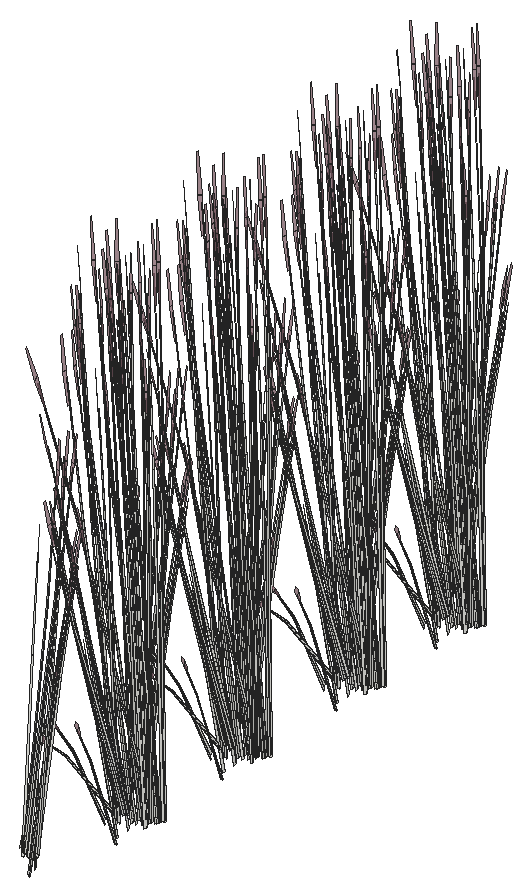
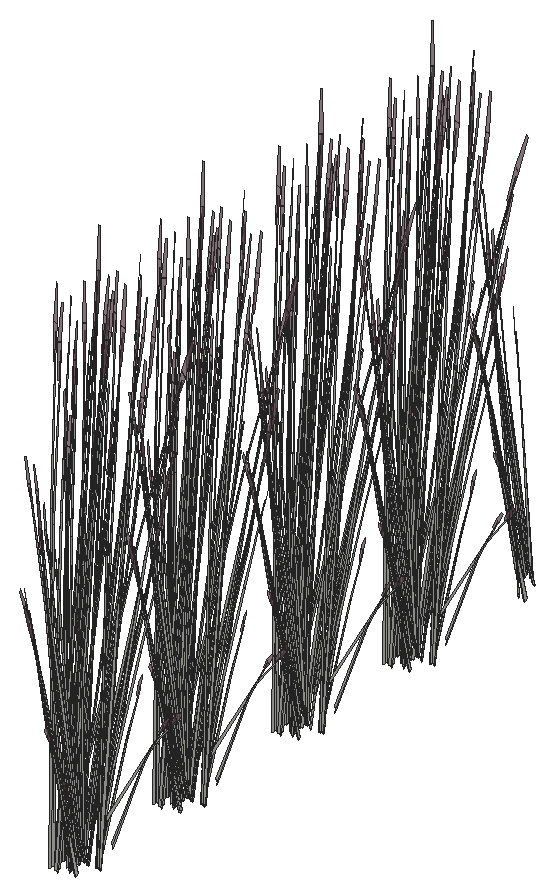
# SketchUp Ruby script. Lengths in inches.
U = 1.inch
M = Sketchup.active_model
def pt(a) = Geom::Point3d.new(a.map { |v| v * U })
def face(e, loops, mat)
  f = e.add_face(loops[0].map { |a| pt(a) })
  loops[1..].each { |l| e.add_face(l.map { |a| pt(a) }).erase! }
  f.material = f.back_material = mat if mat
  f
end
# faces: each face lists its corners as indices into pts; further lists are holes
def faces(e, pts, list, mat = nil) = list.each { |f| face(e, (f[0].is_a?(Array) ? f : [f]).map { |l| l.map { |i| pts[i] } }, mat) }
# xy, xz, yz: faces in a plane at the given z, y or x. An outline is a flat list of corners, or four numbers for a rectangle; further outlines are holes
def ring(l) = l.size == 4 ? [[l[0], l[1]], [l[2], l[1]], [l[2], l[3]], [l[0], l[3]]] : l.each_slice(2).to_a
def flat(e, list, mat, &to3) = list.each { |f| face(e, (f[0].is_a?(Array) ? f : [f]).map { |l| ring(l).map { |u, v| to3.(u, v) } }, mat) }
def xy(e, z, list, mat = nil) = flat(e, list, mat) { |x, y| [x, y, z] }
def xz(e, y, list, mat = nil) = flat(e, list, mat) { |x, z| [x, y, z] }
def yz(e, x, list, mat = nil) = flat(e, list, mat) { |y, z| [x, y, z] }
def lines(e, pts, list) = list.each { |a, b| e.add_line(pt(pts[a]), pt(pts[b])) }
# prism: a flat outline (further loops are holes) pulled along v
def prism(e, loops, v, mat = nil)
  f = face(e, loops, mat); d = Geom::Vector3d.new(v.map { |x| x * U })
  f.pushpull(f.normal.samedirection?(d) ? d.length : -d.length)
end
def box(e, o, s, mat = nil) = prism(e, [[o, [o[0] + s[0], o[1], o[2]], [o[0] + s[0], o[1] + s[1], o[2]], [o[0], o[1] + s[1], o[2]]]], [0, 0, s[2]], mat)
def at(x, y, z, deg = 0) = Geom::Transformation.translation(pt([x, y, z])) * Geom::Transformation.rotation(ORIGIN, Z_AXIS, deg.degrees)
def axes(o, x, y, z) = Geom::Transformation.new([*x, 0, *y, 0, *z, 0, *pt(o).to_a, 1])
def part(name) = M.definitions.add(name)
# library, detail: a bought-in or finely detailed component or shape, given as its bounding box
def library(name, o, s) = part(name).tap { |d| box(d.entities, o, s) }
def detail(e, o, s) = box(e.add_group.entities, o, s)
def put(e, d, t, mat = nil) = e.add_instance(d, t).tap { |i| i.material = mat if mat }
def group(e, t, mat = nil) = e.add_group.tap { |g| g.transformation = t; g.material = mat if mat }.entities
root = M.entities
M.materials.add("LightPink_Translucent").color = [144, 107, 117]
M.materials["LightPink_Translucent"].alpha = 0.75
c1 = part("blade")
p = [[2.15,0.21,22],[0,0.17,0],[0.09,0.45,0],[2.18,0.31,22],[2.29,0.31,22],[0.38,0.45,0],
  [2.48,0.24,33],[2.49,0.24,33],[2.48,0.22,33]]
faces(c1.entities,p,[[0,1,2,3],[4,5,2,3],[6,3,4,7],[8,0,3,6]])
c2 = part("seeds")
p = [[0.3,-0.1,1.38],[-0.01,-0.03,1.59],[-0.01,-0.03,0.03],[0.14,-0.07,-0.07],[0.29,-0.03,3],[0.15,0.01,3.11]]
faces(c2.entities,p,[[0,1,2,3],[1,0,4,5]],"LightPink_Translucent")
c3 = part("blade with seeds")
put(c3.entities,c1,at(0,0,0))
put(c3.entities,c2,axes([2.4,0.25,30.99],[1.5799,-0.05474,1.17369],[-0.12525,1.92788,0.29478],[-0.07173,-0.02425,1.56792]))
put(root,c3,axes([340.43,150.67,657.88],[-0.40605,-0.0193,0.05273],[0.01113,-0.29147,0.41509],[-0.04249,0.11165,0.63295]))
put(root,c3,axes([340.43,163.31,657.88],[-0.40605,-0.0193,0.05273],[0.01113,-0.29147,0.41509],[-0.04249,0.11165,0.63295]))
put(root,c3,axes([340.43,176.78,657.88],[-0.40605,-0.0193,0.05273],[0.01113,-0.29147,0.41509],[-0.04249,0.11165,0.63295]))
put(root,c3,axes([340.43,188.65,657.88],[-0.40605,-0.0193,0.05273],[0.01113,-0.29147,0.41509],[-0.04249,0.11165,0.63295]))
put(root,c3,axes([340.5625,137.6875,657.71],[-0.33433,0.21811,-0.29039],[-0.31649,-0.24905,0.3749],[-0.04815,0.12654,0.71734]))
put(root,c3,axes([340.5625,150.78,657.71],[-0.33433,0.21811,-0.29039],[-0.31649,-0.24905,0.3749],[-0.04815,0.12654,0.71734]))
put(root,c3,axes([340.5625,163.42,657.71],[-0.33433,0.21811,-0.29039],[-0.31649,-0.24905,0.3749],[-0.04815,0.12654,0.71734]))
put(root,c3,axes([340.5625,176.9,657.71],[-0.33433,0.21811,-0.29039],[-0.31649,-0.24905,0.3749],[-0.04815,0.12654,0.71734]))
put(root,c3,axes([340.5625,188.76,657.71],[-0.33433,0.21811,-0.29039],[-0.31649,-0.24905,0.3749],[-0.04815,0.12654,0.71734]))
put(root,c3,axes([342.27,150.13,655.6875],[-0.33282,0.31137,-0.51129],[-0.41344,-0.28235,-0.13419],[-0.13336,0.07767,1.12859]))
put(root,c3,axes([342.27,162.77,655.6875],[-0.33282,0.31137,-0.51129],[-0.41344,-0.28235,-0.13419],[-0.13336,0.07767,1.12859]))
put(root,c3,axes([342.27,176.24,655.6875],[-0.33282,0.31137,-0.51129],[-0.41344,-0.28235,-0.13419],[-0.13336,0.07767,1.12859]))
put(root,c3,axes([342.27,188.1,655.6875],[-0.33282,0.31137,-0.51129],[-0.41344,-0.28235,-0.13419],[-0.13336,0.07767,1.12859]))
put(root,c3,axes([341.42,147.81,658.14],[0.07631,0.33368,0.29039],[-0.43626,0.08811,-0.3749],[-0.11718,-0.09562,0.71734]))
put(root,c3,axes([341.42,160.45,658.14],[0.07631,0.33368,0.29039],[-0.43626,0.08811,-0.3749],[-0.11718,-0.09562,0.71734]))
put(root,c3,axes([341.42,173.93,658.14],[0.07631,0.33368,0.29039],[-0.43626,0.08811,-0.3749],[-0.11718,-0.09562,0.71734]))
put(root,c3,axes([341.42,185.79,658.14],[0.07631,0.33368,0.29039],[-0.43626,0.08811,-0.3749],[-0.11718,-0.09562,0.71734]))
put(root,c3,axes([339.37,138.46,657.86],[0.05606,-0.02501,1.45454],[0.46332,0.16636,-0.13744],[-0.01089,0.13852,0.2574]))
put(root,c3,axes([339.37,151.56,657.86],[0.05606,-0.02501,1.45454],[0.46332,0.16636,-0.13744],[-0.01089,0.13852,0.2574]))
put(root,c3,axes([339.37,164.19,657.86],[0.05606,-0.02501,1.45454],[0.46332,0.16636,-0.13744],[-0.01089,0.13852,0.2574]))
put(root,c3,axes([339.37,177.67,657.86],[0.05606,-0.02501,1.45454],[0.46332,0.16636,-0.13744],[-0.01089,0.13852,0.2574]))
put(root,c3,axes([339.37,189.53,657.86],[0.05606,-0.02501,1.45454],[0.46332,0.16636,-0.13744],[-0.01089,0.13852,0.2574]))
put(root,c3,axes([340.42,149.11,655.91],[-0.45961,0.34828,0.2522],[-0.45989,-0.34462,-0.29923],[-0.01605,-0.09891,1.35206]))
put(root,c3,axes([340.42,161.74,655.91],[-0.45961,0.34828,0.2522],[-0.45989,-0.34462,-0.29923],[-0.01605,-0.09891,1.35206]))
put(root,c3,axes([340.42,175.22,655.91],[-0.45961,0.34828,0.2522],[-0.45989,-0.34462,-0.29923],[-0.01605,-0.09891,1.35206]))
put(root,c3,axes([340.42,187.08,655.91],[-0.45961,0.34828,0.2522],[-0.45989,-0.34462,-0.29923],[-0.01605,-0.09891,1.35206]))
put(root,c3,axes([342.3125,150.07,656.73],[0.427,0.16705,1.24034],[-0.41831,0.35988,0.49049],[-0.18737,-0.21329,1.03981]))
put(root,c3,axes([342.3125,162.71,656.73],[0.427,0.16705,1.24034],[-0.41831,0.35988,0.49049],[-0.18737,-0.21329,1.03981]))
put(root,c3,axes([342.3125,176.18,656.73],[0.427,0.16705,1.24034],[-0.41831,0.35988,0.49049],[-0.18737,-0.21329,1.03981]))
put(root,c3,axes([342.3125,188.04,656.73],[0.427,0.16705,1.24034],[-0.41831,0.35988,0.49049],[-0.18737,-0.21329,1.03981]))
put(root,c3,axes([340.68,147.04,656.27],[0.25775,0.14418,0.94186],[-0.37538,0.08667,0.69201],[-0.08032,-0.11081,0.20745]))
put(root,c3,axes([340.68,159.68,656.27],[0.25775,0.14418,0.94186],[-0.37538,0.08667,0.69201],[-0.08032,-0.11081,0.20745]))
put(root,c3,axes([340.68,173.15,656.27],[0.25775,0.14418,0.94186],[-0.37538,0.08667,0.69201],[-0.08032,-0.11081,0.20745]))
put(root,c3,axes([340.68,185.02,656.27],[0.25775,0.14418,0.94186],[-0.37538,0.08667,0.69201],[-0.08032,-0.11081,0.20745]))
put(root,c3,axes([342.5,149.95,656.02],[-0.48249,-0.33343,-0.20658],[0.406,-0.37441,0.45206],[-0.12993,0.039,1.37937]))
put(root,c3,axes([342.5,162.59,656.02],[-0.48249,-0.33343,-0.20658],[0.406,-0.37441,0.45206],[-0.12993,0.039,1.37937]))
put(root,c3,axes([342.5,176.07,656.02],[-0.48249,-0.33343,-0.20658],[0.406,-0.37441,0.45206],[-0.12993,0.039,1.37937]))
put(root,c3,axes([342.5,187.93,656.02],[-0.48249,-0.33343,-0.20658],[0.406,-0.37441,0.45206],[-0.12993,0.039,1.37937]))
put(root,c3,axes([341.625,149.63,655.8125],[-0.29683,-0.34771,-0.36686],[0.44961,-0.24485,0.17656],[-0.09606,-0.04302,1.17788]))
put(root,c3,axes([341.625,162.27,655.8125],[-0.29683,-0.34771,-0.36686],[0.44961,-0.24485,0.17656],[-0.09606,-0.04302,1.17788]))
put(root,c3,axes([341.625,175.75,655.8125],[-0.29683,-0.34771,-0.36686],[0.44961,-0.24485,0.17656],[-0.09606,-0.04302,1.17788]))
put(root,c3,axes([341.625,187.61,655.8125],[-0.29683,-0.34771,-0.36686],[0.44961,-0.24485,0.17656],[-0.09606,-0.04302,1.17788]))
put(root,c3,axes([340.78,137.46,658.38],[-0.01286,0.38319,-0.64665],[-0.54141,-0.02574,0.07804],[-0.05714,0.16234,0.91476]))
put(root,c3,axes([340.78,150.55,658.38],[-0.01286,0.38319,-0.64665],[-0.54141,-0.02574,0.07804],[-0.05714,0.16234,0.91476]))
put(root,c3,axes([340.78,163.1875,658.38],[-0.01286,0.38319,-0.64665],[-0.54141,-0.02574,0.07804],[-0.05714,0.16234,0.91476]))
put(root,c3,axes([340.78,176.67,658.38],[-0.01286,0.38319,-0.64665],[-0.54141,-0.02574,0.07804],[-0.05714,0.16234,0.91476]))
put(root,c3,axes([340.78,188.53,658.38],[-0.01286,0.38319,-0.64665],[-0.54141,-0.02574,0.07804],[-0.05714,0.16234,0.91476]))
put(root,c3,axes([340.77,138.54,656.27],[-0.01279,-0.24632,0.94186],[0.31954,0.17569,0.69201],[-0.06284,0.11741,0.20745]))
put(root,c3,axes([340.77,151.63,656.27],[-0.01279,-0.24632,0.94186],[0.31954,0.17569,0.69201],[-0.06284,0.11741,0.20745]))
put(root,c3,axes([340.77,164.27,656.27],[-0.01279,-0.24632,0.94186],[0.31954,0.17569,0.69201],[-0.06284,0.11741,0.20745]))
put(root,c3,axes([340.77,177.74,656.27],[-0.01279,-0.24632,0.94186],[0.31954,0.17569,0.69201],[-0.06284,0.11741,0.20745]))
put(root,c3,axes([340.77,189.6,656.27],[-0.01279,-0.24632,0.94186],[0.31954,0.17569,0.69201],[-0.06284,0.11741,0.20745]))
put(root,c3,axes([341.22,147.42,658.18],[0.55043,-0.10648,0.44086],[0.09553,0.41768,0.3635],[-0.12945,-0.1231,0.91224]))
put(root,c3,axes([341.22,160.06,658.18],[0.55043,-0.10648,0.44086],[0.09553,0.41768,0.3635],[-0.12945,-0.1231,0.91224]))
put(root,c3,axes([341.22,173.53,658.18],[0.55043,-0.10648,0.44086],[0.09553,0.41768,0.3635],[-0.12945,-0.1231,0.91224]))
put(root,c3,axes([341.22,185.39,658.18],[0.55043,-0.10648,0.44086],[0.09553,0.41768,0.3635],[-0.12945,-0.1231,0.91224]))
put(root,c3,axes([342.26,149.88,655.8125],[-0.53657,0.02557,-0.36686],[-0.04852,-0.4245,0.17656],[-0.09606,0.04302,1.17788]))
put(root,c3,axes([342.26,162.52,655.8125],[-0.53657,0.02557,-0.36686],[-0.04852,-0.4245,0.17656],[-0.09606,0.04302,1.17788]))
put(root,c3,axes([342.26,176,655.8125],[-0.53657,0.02557,-0.36686],[-0.04852,-0.4245,0.17656],[-0.09606,0.04302,1.17788]))
put(root,c3,axes([342.26,187.86,655.8125],[-0.53657,0.02557,-0.36686],[-0.04852,-0.4245,0.17656],[-0.09606,0.04302,1.17788]))
put(root,c3,axes([341.35,147.51,657.88],[0.22457,-0.26316,0.05273],[0.3198,0.15321,0.41509],[-0.10339,-0.08437,0.63295]))
put(root,c3,axes([341.35,160.15,657.88],[0.22457,-0.26316,0.05273],[0.3198,0.15321,0.41509],[-0.10339,-0.08437,0.63295]))
put(root,c3,axes([341.35,173.62,657.88],[0.22457,-0.26316,0.05273],[0.3198,0.15321,0.41509],[-0.10339,-0.08437,0.63295]))
put(root,c3,axes([341.35,185.48,657.88],[0.22457,-0.26316,0.05273],[0.3198,0.15321,0.41509],[-0.10339,-0.08437,0.63295]))
put(root,c3,axes([341.23,150.59,656.03],[0.46245,0.20713,0.40713],[-0.27641,0.37142,0],[-0.10533,-0.04718,1.29153]))
put(root,c3,axes([341.23,163.23,656.03],[0.46245,0.20713,0.40713],[-0.27641,0.37142,0],[-0.10533,-0.04718,1.29153]))
put(root,c3,axes([341.23,176.71,656.03],[0.46245,0.20713,0.40713],[-0.27641,0.37142,0],[-0.10533,-0.04718,1.29153]))
put(root,c3,axes([341.23,188.57,656.03],[0.46245,0.20713,0.40713],[-0.27641,0.37142,0],[-0.10533,-0.04718,1.29153]))
put(root,c3,axes([340.6,138,656.76],[0.01086,-0.21386,1.26563],[0.48828,0.11296,0.1749],[-0.04231,0.22792,0.59763]))
put(root,c3,axes([340.6,151.09,656.76],[0.01086,-0.21386,1.26563],[0.48828,0.11296,0.1749],[-0.04231,0.22792,0.59763]))
put(root,c3,axes([340.6,163.73,656.76],[0.01086,-0.21386,1.26563],[0.48828,0.11296,0.1749],[-0.04231,0.22792,0.59763]))
put(root,c3,axes([340.6,177.21,656.76],[0.01086,-0.21386,1.26563],[0.48828,0.11296,0.1749],[-0.04231,0.22792,0.59763]))
put(root,c3,axes([340.6,189.07,656.76],[0.01086,-0.21386,1.26563],[0.48828,0.11296,0.1749],[-0.04231,0.22792,0.59763]))
put(root,c3,axes([341.67,149.83,656],[0.13096,-0.49088,-0.19212],[0.62096,0.08557,0.42042],[-0.1085,-0.06779,1.28281]))
put(root,c3,axes([341.67,162.47,656],[0.13096,-0.49088,-0.19212],[0.62096,0.08557,0.42042],[-0.1085,-0.06779,1.28281]))
put(root,c3,axes([341.67,175.95,656],[0.13096,-0.49088,-0.19212],[0.62096,0.08557,0.42042],[-0.1085,-0.06779,1.28281]))
put(root,c3,axes([341.67,187.81,656],[0.13096,-0.49088,-0.19212],[0.62096,0.08557,0.42042],[-0.1085,-0.06779,1.28281]))
put(root,c3,axes([341.89,149.95,656.15],[-0.09532,0.36971,0.11873],[-0.46572,-0.06418,-0.33905],[-0.08476,-0.03796,1.0393]))
put(root,c3,axes([341.89,162.59,656.15],[-0.09532,0.36971,0.11873],[-0.46572,-0.06418,-0.33905],[-0.08476,-0.03796,1.0393]))
put(root,c3,axes([341.89,176.0625,656.15],[-0.09532,0.36971,0.11873],[-0.46572,-0.06418,-0.33905],[-0.08476,-0.03796,1.0393]))
put(root,c3,axes([341.89,187.92,656.15],[-0.09532,0.36971,0.11873],[-0.46572,-0.06418,-0.33905],[-0.08476,-0.03796,1.0393]))
put(root,c3,axes([341.84,146.73,657.87],[-0.07558,-0.05808,1.43454],[-0.50436,0.03682,-0.22687],[-0.08049,-0.13892,0.11505]))
put(root,c3,axes([341.84,159.36,657.87],[-0.07558,-0.05808,1.43454],[-0.50436,0.03682,-0.22687],[-0.08049,-0.13892,0.11505]))
put(root,c3,axes([341.84,172.84,657.87],[-0.07558,-0.05808,1.43454],[-0.50436,0.03682,-0.22687],[-0.08049,-0.13892,0.11505]))
put(root,c3,axes([341.84,184.7,657.87],[-0.07558,-0.05808,1.43454],[-0.50436,0.03682,-0.22687],[-0.08049,-0.13892,0.11505]))
put(root,c3,axes([342.82,150.98,655.65],[-0.46245,0.20713,-0.40713],[-0.27641,-0.37142,0],[-0.10533,0.04718,1.29153]))
put(root,c3,axes([342.82,163.62,655.65],[-0.46245,0.20713,-0.40713],[-0.27641,-0.37142,0],[-0.10533,0.04718,1.29153]))
put(root,c3,axes([342.82,177.09,655.65],[-0.46245,0.20713,-0.40713],[-0.27641,-0.37142,0],[-0.10533,0.04718,1.29153]))
put(root,c3,axes([342.82,188.95,655.65],[-0.46245,0.20713,-0.40713],[-0.27641,-0.37142,0],[-0.10533,0.04718,1.29153]))
put(root,c3,axes([340.08,148.91,655.65],[0,-0.41426,-0.40713],[0.55282,0,0],[0,-0.09435,1.29153]))
put(root,c3,axes([340.08,161.55,655.65],[0,-0.41426,-0.40713],[0.55282,0,0],[0,-0.09435,1.29153]))
put(root,c3,axes([340.08,175.03,655.65],[0,-0.41426,-0.40713],[0.55282,0,0],[0,-0.09435,1.29153]))
put(root,c3,axes([340.08,186.89,655.65],[0,-0.41426,-0.40713],[0.55282,0,0],[0,-0.09435,1.29153]))
put(root,c3,axes([340.32,149.3,656.03],[0,0.41426,0.40713],[-0.55282,0,0],[0,-0.09435,1.29153]))
put(root,c3,axes([340.32,161.9375,656.03],[0,0.41426,0.40713],[-0.55282,0,0],[0,-0.09435,1.29153]))
put(root,c3,axes([340.32,175.41,656.03],[0,0.41426,0.40713],[-0.55282,0,0],[0,-0.09435,1.29153]))
put(root,c3,axes([340.32,187.27,656.03],[0,0.41426,0.40713],[-0.55282,0,0],[0,-0.09435,1.29153]))
put(root,c3,axes([342.85,150.87,655.8],[-0.30508,-0.41657,-0.04217],[0.51685,-0.2315,0.42318],[-0.12736,0.03966,1.34177]))
put(root,c3,axes([342.85,163.5,655.8],[-0.30508,-0.41657,-0.04217],[0.51685,-0.2315,0.42318],[-0.12736,0.03966,1.34177]))
put(root,c3,axes([342.85,176.98,655.8],[-0.30508,-0.41657,-0.04217],[0.51685,-0.2315,0.42318],[-0.12736,0.03966,1.34177]))
put(root,c3,axes([342.85,188.84,655.8],[-0.30508,-0.41657,-0.04217],[0.51685,-0.2315,0.42318],[-0.12736,0.03966,1.34177]))
put(root,c3,axes([340.89,137.59,658.1],[0.35372,0.27835,-0.4651],[-0.37366,0.24377,-0.36026],[-0.05382,0.14142,0.88993]))
put(root,c3,axes([340.89,150.68,658.1],[0.35372,0.27835,-0.4651],[-0.37366,0.24377,-0.36026],[-0.05382,0.14142,0.88993]))
put(root,c3,axes([340.89,163.32,658.1],[0.35372,0.27835,-0.4651],[-0.37366,0.24377,-0.36026],[-0.05382,0.14142,0.88993]))
put(root,c3,axes([340.89,176.79,658.1],[0.35372,0.27835,-0.4651],[-0.37366,0.24377,-0.36026],[-0.05382,0.14142,0.88993]))
put(root,c3,axes([340.89,188.65,658.1],[0.35372,0.27835,-0.4651],[-0.37366,0.24377,-0.36026],[-0.05382,0.14142,0.88993]))
put(root,c3,axes([342.71,150.8125,655.66],[-0.46099,-0.1025,-0.25402],[0.11607,-0.36097,0.25402],[-0.09293,0.04163,1.13959]))
put(root,c3,axes([342.71,163.45,655.66],[-0.46099,-0.1025,-0.25402],[0.11607,-0.36097,0.25402],[-0.09293,0.04163,1.13959]))
put(root,c3,axes([342.71,176.93,655.66],[-0.46099,-0.1025,-0.25402],[0.11607,-0.36097,0.25402],[-0.09293,0.04163,1.13959]))
put(root,c3,axes([342.71,188.79,655.66],[-0.46099,-0.1025,-0.25402],[0.11607,-0.36097,0.25402],[-0.09293,0.04163,1.13959]))
put(root,c3,axes([340.74,150.47,658.14],[0.33433,-0.21811,0.29039],[0.31649,0.24905,-0.3749],[-0.04815,0.12654,0.71734]))
put(root,c3,axes([340.74,163.11,658.14],[0.33433,-0.21811,0.29039],[0.31649,0.24905,-0.3749],[-0.04815,0.12654,0.71734]))
put(root,c3,axes([340.74,176.59,658.14],[0.33433,-0.21811,0.29039],[0.31649,0.24905,-0.3749],[-0.04815,0.12654,0.71734]))
put(root,c3,axes([340.74,188.45,658.14],[0.33433,-0.21811,0.29039],[0.31649,0.24905,-0.3749],[-0.04815,0.12654,0.71734]))
put(root,c3,axes([341.53,149.39,656.1875],[-0.55647,-0.19766,-0.23858],[0.26794,-0.4172,-0.41002],[-0.01749,-0.10243,1.3096]))
put(root,c3,axes([341.53,162.03,656.1875],[-0.55647,-0.19766,-0.23858],[0.26794,-0.4172,-0.41002],[-0.01749,-0.10243,1.3096]))
put(root,c3,axes([341.53,175.51,656.1875],[-0.55647,-0.19766,-0.23858],[0.26794,-0.4172,-0.41002],[-0.01749,-0.10243,1.3096]))
put(root,c3,axes([341.53,187.37,656.1875],[-0.55647,-0.19766,-0.23858],[0.26794,-0.4172,-0.41002],[-0.01749,-0.10243,1.3096]))
put(root,c3,axes([342.98,149.27,656.33],[-0.0135,-0.39004,1.15843],[0.61089,0.10111,0.49049],[-0.14449,0.21343,1.09347]))
put(root,c3,axes([342.98,161.91,656.33],[-0.0135,-0.39004,1.15843],[0.61089,0.10111,0.49049],[-0.14449,0.21343,1.09347]))
put(root,c3,axes([342.98,175.39,656.33],[-0.0135,-0.39004,1.15843],[0.61089,0.10111,0.49049],[-0.14449,0.21343,1.09347]))
put(root,c3,axes([342.98,187.25,656.33],[-0.0135,-0.39004,1.15843],[0.61089,0.10111,0.49049],[-0.14449,0.21343,1.09347]))
put(root,c3,axes([340.52,137.4375,658.43],[0.54305,0.02053,-0.11068],[-0.01484,0.38862,-0.61434],[-0.03772,0.14967,0.93347]))
put(root,c3,axes([340.52,150.53,658.43],[0.54305,0.02053,-0.11068],[-0.01484,0.38862,-0.61434],[-0.03772,0.14967,0.93347]))
put(root,c3,axes([340.52,163.17,658.43],[0.54305,0.02053,-0.11068],[-0.01484,0.38862,-0.61434],[-0.03772,0.14967,0.93347]))
put(root,c3,axes([340.52,176.65,658.43],[0.54305,0.02053,-0.11068],[-0.01484,0.38862,-0.61434],[-0.03772,0.14967,0.93347]))
put(root,c3,axes([340.52,188.51,658.43],[0.54305,0.02053,-0.11068],[-0.01484,0.38862,-0.61434],[-0.03772,0.14967,0.93347]))
put(root,c3,axes([340.51,138,656.31],[0.44888,-0.07336,0.05336],[0.1032,0.29555,-0.7077],[-0.02846,0.14961,0.63435]))
put(root,c3,axes([340.51,151.1,656.31],[0.44888,-0.07336,0.05336],[0.1032,0.29555,-0.7077],[-0.02846,0.14961,0.63435]))
put(root,c3,axes([340.51,163.73,656.31],[0.44888,-0.07336,0.05336],[0.1032,0.29555,-0.7077],[-0.02846,0.14961,0.63435]))
put(root,c3,axes([340.51,177.21,656.31],[0.44888,-0.07336,0.05336],[0.1032,0.29555,-0.7077],[-0.02846,0.14961,0.63435]))
put(root,c3,axes([340.51,189.07,656.31],[0.44888,-0.07336,0.05336],[0.1032,0.29555,-0.7077],[-0.02846,0.14961,0.63435]))
put(root,c3,axes([342.63,149.77,656.1875],[0.05758,0.4727,-0.23858],[-0.59969,0.02858,-0.41002],[-0.1056,0.06296,1.3096]))
put(root,c3,axes([342.63,162.4,656.1875],[0.05758,0.4727,-0.23858],[-0.59969,0.02858,-0.41002],[-0.1056,0.06296,1.3096]))
put(root,c3,axes([342.63,175.88,656.1875],[0.05758,0.4727,-0.23858],[-0.59969,0.02858,-0.41002],[-0.1056,0.06296,1.3096]))
put(root,c3,axes([342.63,187.74,656.1875],[0.05758,0.4727,-0.23858],[-0.59969,0.02858,-0.41002],[-0.1056,0.06296,1.3096]))
put(root,c3,axes([341.28,148.97,655.72],[-0.20292,-0.42481,-0.57265],[0.58453,-0.15299,-0.1503],[-0.02243,-0.14385,1.26402]))
put(root,c3,axes([341.28,161.61,655.72],[-0.20292,-0.42481,-0.57265],[0.58453,-0.15299,-0.1503],[-0.02243,-0.14385,1.26402]))
put(root,c3,axes([341.28,175.09,655.72],[-0.20292,-0.42481,-0.57265],[0.58453,-0.15299,-0.1503],[-0.02243,-0.14385,1.26402]))
put(root,c3,axes([341.28,186.95,655.72],[-0.20292,-0.42481,-0.57265],[0.58453,-0.15299,-0.1503],[-0.02243,-0.14385,1.26402]))
put(root,c3,axes([342.61,147.62,658.13],[-0.48353,0.19287,-0.09971],[-0.23761,-0.34232,-0.55346],[-0.0638,-0.14425,0.84097]))
put(root,c3,axes([342.61,160.26,658.13],[-0.48353,0.19287,-0.09971],[-0.23761,-0.34232,-0.55346],[-0.0638,-0.14425,0.84097]))
put(root,c3,axes([342.61,173.74,658.13],[-0.48353,0.19287,-0.09971],[-0.23761,-0.34232,-0.55346],[-0.0638,-0.14425,0.84097]))
put(root,c3,axes([342.61,185.6,658.13],[-0.48353,0.19287,-0.09971],[-0.23761,-0.34232,-0.55346],[-0.0638,-0.14425,0.84097]))
put(root,c3,axes([342.19,147.64,657.84],[-0.48573,-0.10385,-0.41901],[0.16649,-0.35605,-0.32456],[-0.04454,-0.14335,0.80174]))
put(root,c3,axes([342.19,160.28,657.84],[-0.48573,-0.10385,-0.41901],[0.16649,-0.35605,-0.32456],[-0.04454,-0.14335,0.80174]))
put(root,c3,axes([342.19,173.76,657.84],[-0.48573,-0.10385,-0.41901],[0.16649,-0.35605,-0.32456],[-0.04454,-0.14335,0.80174]))
put(root,c3,axes([342.19,185.62,657.84],[-0.48573,-0.10385,-0.41901],[0.16649,-0.35605,-0.32456],[-0.04454,-0.14335,0.80174]))
put(root,c3,axes([341.3,137.1875,657.18],[-0.01209,-0.159,1.40529],[0.52417,0.10548,0.11363],[-0.03242,0.22659,0.60075]))
put(root,c3,axes([341.3,150.28,657.18],[-0.01209,-0.159,1.40529],[0.52417,0.10548,0.11363],[-0.03242,0.22659,0.60075]))
put(root,c3,axes([341.3,162.92,657.18],[-0.01209,-0.159,1.40529],[0.52417,0.10548,0.11363],[-0.03242,0.22659,0.60075]))
put(root,c3,axes([341.3,176.39,657.18],[-0.01209,-0.159,1.40529],[0.52417,0.10548,0.11363],[-0.03242,0.22659,0.60075]))
put(root,c3,axes([341.3,188.26,657.18],[-0.01209,-0.159,1.40529],[0.52417,0.10548,0.11363],[-0.03242,0.22659,0.60075]))
put(root,c3,axes([340.32,148.92,655.66],[0.34492,-0.25847,-0.25402],[0.34492,0.25847,0.25402],[0,-0.08325,1.13959]))
put(root,c3,axes([340.32,161.5625,655.66],[0.34492,-0.25847,-0.25402],[0.34492,0.25847,0.25402],[0,-0.08325,1.13959]))
put(root,c3,axes([340.32,175.04,655.66],[0.34492,-0.25847,-0.25402],[0.34492,0.25847,0.25402],[0,-0.08325,1.13959]))
put(root,c3,axes([340.32,186.9,655.66],[0.34492,-0.25847,-0.25402],[0.34492,0.25847,0.25402],[0,-0.08325,1.13959]))
put(root,c3,axes([341.875,147.25,655.74],[-0.34145,0.23766,-0.03192],[-0.31287,-0.26029,-0.14473],[-0.02203,-0.07375,0.47736]))
put(root,c3,axes([341.875,159.89,655.74],[-0.34145,0.23766,-0.03192],[-0.31287,-0.26029,-0.14473],[-0.02203,-0.07375,0.47736]))
put(root,c3,axes([341.875,173.37,655.74],[-0.34145,0.23766,-0.03192],[-0.31287,-0.26029,-0.14473],[-0.02203,-0.07375,0.47736]))
put(root,c3,axes([341.875,185.23,655.74],[-0.34145,0.23766,-0.03192],[-0.31287,-0.26029,-0.14473],[-0.02203,-0.07375,0.47736]))
put(root,c3,axes([341.74,149.6,655.9375],[0.62452,0.08728,0.37519],[-0.1271,0.49295,0.14723],[-0.09127,-0.0476,1.30262]))
put(root,c3,axes([341.74,162.23,655.9375],[0.62452,0.08728,0.37519],[-0.1271,0.49295,0.14723],[-0.09127,-0.0476,1.30262]))
put(root,c3,axes([341.74,175.71,655.9375],[0.62452,0.08728,0.37519],[-0.1271,0.49295,0.14723],[-0.09127,-0.0476,1.30262]))
put(root,c3,axes([341.74,187.57,655.9375],[0.62452,0.08728,0.37519],[-0.1271,0.49295,0.14723],[-0.09127,-0.0476,1.30262]))
put(root,c3,axes([341.58,149.51,656.23],[-0.23974,0.37328,0.36686],[-0.49814,-0.17965,-0.17656],[0,-0.08605,1.17788]))
put(root,c3,axes([341.58,162.14,656.23],[-0.23974,0.37328,0.36686],[-0.49814,-0.17965,-0.17656],[0,-0.08605,1.17788]))
put(root,c3,axes([341.58,175.62,656.23],[-0.23974,0.37328,0.36686],[-0.49814,-0.17965,-0.17656],[0,-0.08605,1.17788]))
put(root,c3,axes([341.58,187.48,656.23],[-0.23974,0.37328,0.36686],[-0.49814,-0.17965,-0.17656],[0,-0.08605,1.17788]))
put(root,c3,axes([342.37,147.71,658.08],[-0.23583,-0.33684,-0.58257],[0.48546,-0.18772,0.0703],[-0.05515,-0.16275,0.8241]))
put(root,c3,axes([342.37,160.35,658.08],[-0.23583,-0.33684,-0.58257],[0.48546,-0.18772,0.0703],[-0.05515,-0.16275,0.8241]))
put(root,c3,axes([342.37,173.82,658.08],[-0.23583,-0.33684,-0.58257],[0.48546,-0.18772,0.0703],[-0.05515,-0.16275,0.8241]))
put(root,c3,axes([342.37,185.68,658.08],[-0.23583,-0.33684,-0.58257],[0.48546,-0.18772,0.0703],[-0.05515,-0.16275,0.8241]))
put(root,c3,axes([341.4,150.38,656.03],[0.53096,-0.10995,0.14467],[0.13111,0.40919,0.28771],[-0.04735,-0.05962,1.31534]))
put(root,c3,axes([341.4,163.02,656.03],[0.53096,-0.10995,0.14467],[0.13111,0.40919,0.28771],[-0.04735,-0.05962,1.31534]))
put(root,c3,axes([341.4,176.5,656.03],[0.53096,-0.10995,0.14467],[0.13111,0.40919,0.28771],[-0.04735,-0.05962,1.31534]))
put(root,c3,axes([341.4,188.36,656.03],[0.53096,-0.10995,0.14467],[0.13111,0.40919,0.28771],[-0.04735,-0.05962,1.31534]))
put(root,c3,axes([342.09,150.45,655.8],[-0.49814,-0.18599,0],[0.23974,-0.38645,0],[0,0,1.3342]))
put(root,c3,axes([342.09,163.09,655.8],[-0.49814,-0.18599,0],[0.23974,-0.38645,0],[0,0,1.3342]))
put(root,c3,axes([342.09,176.5625,655.8],[-0.49814,-0.18599,0],[0.23974,-0.38645,0],[0,0,1.3342]))
put(root,c3,axes([342.09,188.42,655.8],[-0.49814,-0.18599,0],[0.23974,-0.38645,0],[0,0,1.3342]))
put(root,c3,axes([342.46,147.76,658.14],[-0.14896,0.31857,0.29039],[-0.4346,-0.09292,-0.3749],[-0.03985,-0.12826,0.71734]))
put(root,c3,axes([342.46,160.4,658.14],[-0.14896,0.31857,0.29039],[-0.4346,-0.09292,-0.3749],[-0.03985,-0.12826,0.71734]))
put(root,c3,axes([342.46,173.87,658.14],[-0.14896,0.31857,0.29039],[-0.4346,-0.09292,-0.3749],[-0.03985,-0.12826,0.71734]))
put(root,c3,axes([342.46,185.73,658.14],[-0.14896,0.31857,0.29039],[-0.4346,-0.09292,-0.3749],[-0.03985,-0.12826,0.71734]))
put(root,c3,axes([343.24,150.91,655.95],[0.30893,0.41511,0],[-0.51685,0.2315,-0.42318],[-0.11772,0.05273,1.34243]))
put(root,c3,axes([343.24,163.55,655.95],[0.30893,0.41511,0],[-0.51685,0.2315,-0.42318],[-0.11772,0.05273,1.34243]))
put(root,c3,axes([343.24,177.03,655.95],[0.30893,0.41511,0],[-0.51685,0.2315,-0.42318],[-0.11772,0.05273,1.34243]))
put(root,c3,axes([343.24,188.89,655.95],[0.30893,0.41511,0],[-0.51685,0.2315,-0.42318],[-0.11772,0.05273,1.34243]))
put(root,c3,axes([341.67,138,658.15],[-0.48688,-0.1083,0.43692],[0.16649,-0.35605,0.36026],[0.02926,0.14002,0.9041]))
put(root,c3,axes([341.67,151.09,658.15],[-0.48688,-0.1083,0.43692],[0.16649,-0.35605,0.36026],[0.02926,0.14002,0.9041]))
put(root,c3,axes([341.67,163.73,658.15],[-0.48688,-0.1083,0.43692],[0.16649,-0.35605,0.36026],[0.02926,0.14002,0.9041]))
put(root,c3,axes([341.67,177.21,658.15],[-0.48688,-0.1083,0.43692],[0.16649,-0.35605,0.36026],[0.02926,0.14002,0.9041]))
put(root,c3,axes([341.67,189.07,658.15],[-0.48688,-0.1083,0.43692],[0.16649,-0.35605,0.36026],[0.02926,0.14002,0.9041]))
put(root,c3,axes([341.54,138.03,657.88],[-0.36409,0.14079,0.05273],[-0.17821,-0.25674,0.41509],[0.03516,0.11317,0.63295]))
put(root,c3,axes([341.54,151.12,657.88],[-0.36409,0.14079,0.05273],[-0.17821,-0.25674,0.41509],[0.03516,0.11317,0.63295]))
put(root,c3,axes([341.54,163.76,657.88],[-0.36409,0.14079,0.05273],[-0.17821,-0.25674,0.41509],[0.03516,0.11317,0.63295]))
put(root,c3,axes([341.54,177.23,657.88],[-0.36409,0.14079,0.05273],[-0.17821,-0.25674,0.41509],[0.03516,0.11317,0.63295]))
put(root,c3,axes([341.54,189.1,657.88],[-0.36409,0.14079,0.05273],[-0.17821,-0.25674,0.41509],[0.03516,0.11317,0.63295]))
put(root,c3,axes([342.98,150.41,656.03],[0.14274,-0.41171,0.14467],[0.52234,0.11651,0.28771],[-0.09023,0.00201,1.31534]))
put(root,c3,axes([342.98,163.04,656.03],[0.14274,-0.41171,0.14467],[0.52234,0.11651,0.28771],[-0.09023,0.00201,1.31534]))
put(root,c3,axes([342.98,176.52,656.03],[0.14274,-0.41171,0.14467],[0.52234,0.11651,0.28771],[-0.09023,0.00201,1.31534]))
put(root,c3,axes([342.98,188.38,656.03],[0.14274,-0.41171,0.14467],[0.52234,0.11651,0.28771],[-0.09023,0.00201,1.31534]))
put(root,c3,axes([342.74,149.86,656.15],[0.36505,0.2489,0.11873],[-0.3045,0.28081,-0.33905],[-0.08476,0.03796,1.0393]))
put(root,c3,axes([342.74,162.5,656.15],[0.36505,0.2489,0.11873],[-0.3045,0.28081,-0.33905],[-0.08476,0.03796,1.0393]))
put(root,c3,axes([342.74,175.97,656.15],[0.36505,0.2489,0.11873],[-0.3045,0.28081,-0.33905],[-0.08476,0.03796,1.0393]))
put(root,c3,axes([342.74,187.84,656.15],[0.36505,0.2489,0.11873],[-0.3045,0.28081,-0.33905],[-0.08476,0.03796,1.0393]))
put(root,c3,axes([342.61,149.55,655.88],[-0.45961,-0.35656,-0.05027],[0.45989,-0.35678,0],[-0.01605,-0.01245,1.43968]))
put(root,c3,axes([342.61,162.19,655.88],[-0.45961,-0.35656,-0.05027],[0.45989,-0.35678,0],[-0.01605,-0.01245,1.43968]))
put(root,c3,axes([342.61,175.67,655.88],[-0.45961,-0.35656,-0.05027],[0.45989,-0.35678,0],[-0.01605,-0.01245,1.43968]))
put(root,c3,axes([342.61,187.53,655.88],[-0.45961,-0.35656,-0.05027],[0.45989,-0.35678,0],[-0.01605,-0.01245,1.43968]))
put(root,c3,axes([342.73,149.68,656.23],[0.53657,-0.02557,0.36686],[0.04852,0.4245,-0.17656],[-0.09606,0.04302,1.17788]))
put(root,c3,axes([342.73,162.3125,656.23],[0.53657,-0.02557,0.36686],[0.04852,0.4245,-0.17656],[-0.09606,0.04302,1.17788]))
put(root,c3,axes([342.73,175.79,656.23],[0.53657,-0.02557,0.36686],[0.04852,0.4245,-0.17656],[-0.09606,0.04302,1.17788]))
put(root,c3,axes([342.73,187.65,656.23],[0.53657,-0.02557,0.36686],[0.04852,0.4245,-0.17656],[-0.09606,0.04302,1.17788]))
put(root,c3,axes([342.86,150.65,655.91],[0.6186,0.13465,0.2522],[-0.15476,0.48129,-0.29923],[-0.10239,0.06024,1.35206]))
put(root,c3,axes([342.86,163.29,655.91],[0.6186,0.13465,0.2522],[-0.15476,0.48129,-0.29923],[-0.10239,0.06024,1.35206]))
put(root,c3,axes([342.86,176.77,655.91],[0.6186,0.13465,0.2522],[-0.15476,0.48129,-0.29923],[-0.10239,0.06024,1.35206]))
put(root,c3,axes([342.86,188.63,655.91],[0.6186,0.13465,0.2522],[-0.15476,0.48129,-0.29923],[-0.10239,0.06024,1.35206]))
put(root,c3,axes([341.96,146.96,655.22],[-0.08288,0.01493,1.44601],[-0.45833,-0.16801,-0.2209],[0.00769,-0.14014,0.2463]))
put(root,c3,axes([341.96,159.6,655.22],[-0.08288,0.01493,1.44601],[-0.45833,-0.16801,-0.2209],[0.00769,-0.14014,0.2463]))
put(root,c3,axes([341.96,173.08,655.22],[-0.08288,0.01493,1.44601],[-0.45833,-0.16801,-0.2209],[0.00769,-0.14014,0.2463]))
put(root,c3,axes([341.96,184.9375,655.22],[-0.08288,0.01493,1.44601],[-0.45833,-0.16801,-0.2209],[0.00769,-0.14014,0.2463]))
put(root,c3,axes([343.13,150.625,656.03],[0.46245,-0.20713,0.40713],[0.27641,0.37142,0],[-0.10533,0.04718,1.29153]))
put(root,c3,axes([343.13,163.26,656.03],[0.46245,-0.20713,0.40713],[0.27641,0.37142,0],[-0.10533,0.04718,1.29153]))
put(root,c3,axes([343.13,176.74,656.03],[0.46245,-0.20713,0.40713],[0.27641,0.37142,0],[-0.10533,0.04718,1.29153]))
put(root,c3,axes([343.13,188.6,656.03],[0.46245,-0.20713,0.40713],[0.27641,0.37142,0],[-0.10533,0.04718,1.29153]))
put(root,c3,axes([342.41,147.42,657.71],[0.14896,-0.31857,-0.29039],[0.4346,0.09292,0.3749],[-0.03985,-0.12826,0.71734]))
